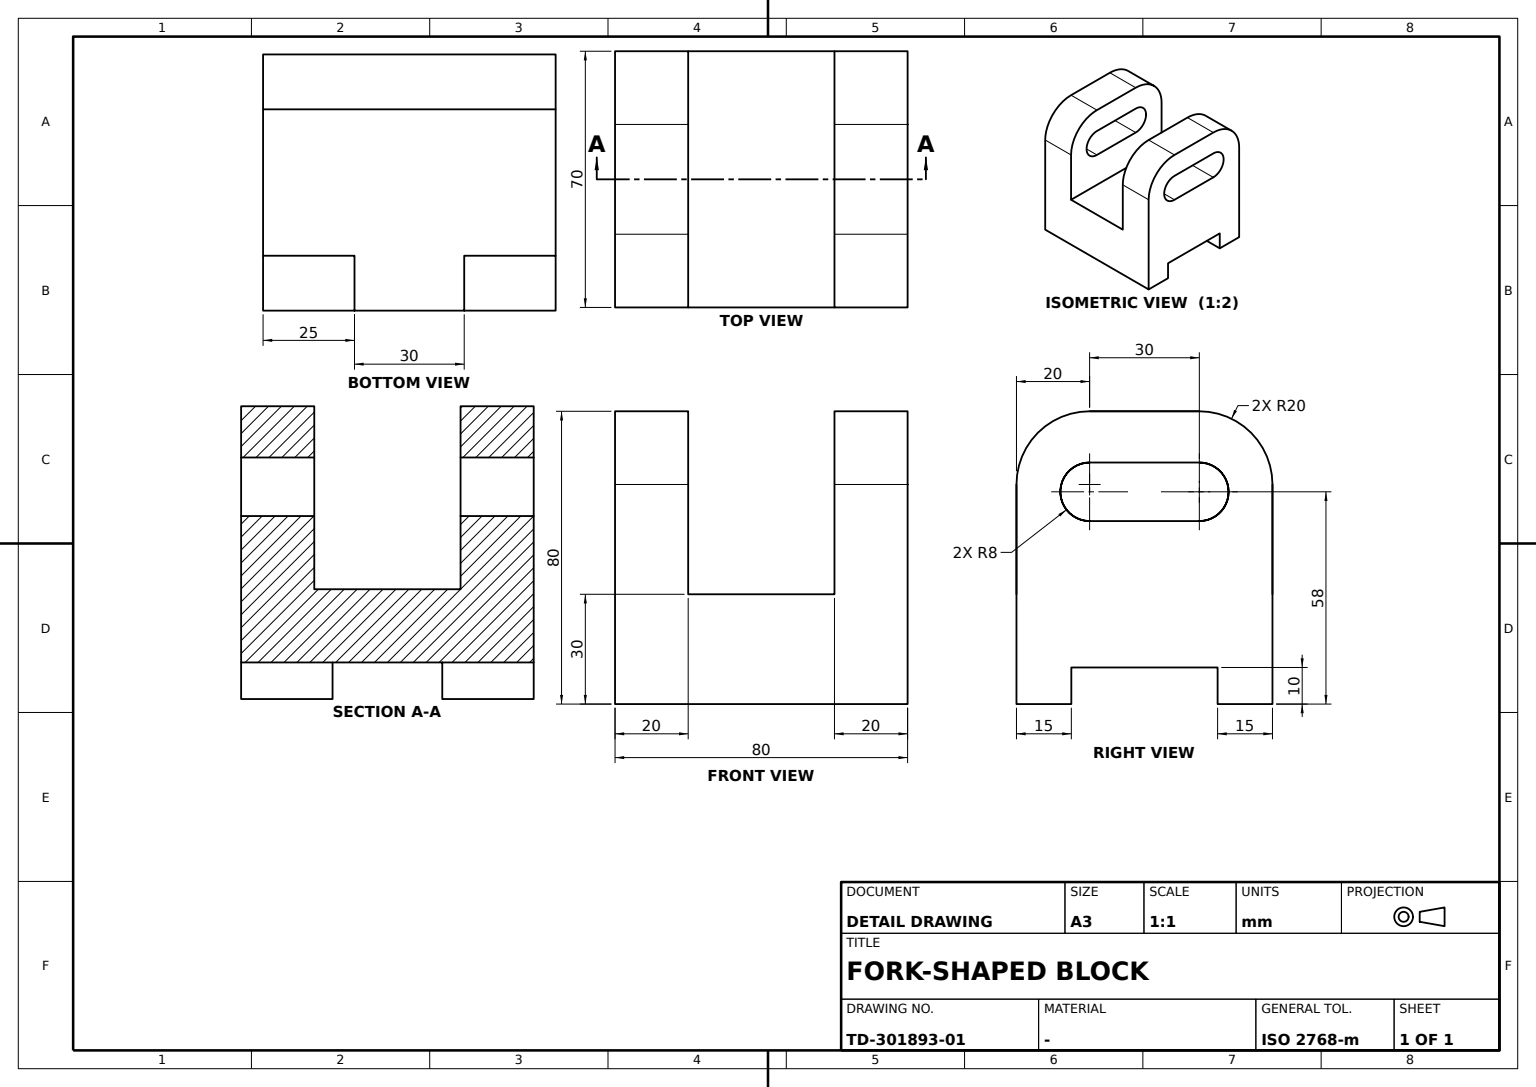
ISO-10303-21;
HEADER;
FILE_DESCRIPTION((''),'2;1');
FILE_NAME('','',(''),(''),'','','');
FILE_SCHEMA(('AUTOMOTIVE_DESIGN'));
ENDSEC;
DATA;
#1=APPLICATION_CONTEXT('');
#2=PRODUCT_CONTEXT('',#1,'mechanical');
#3=PRODUCT('','','',(#2));
#4=PRODUCT_DEFINITION_FORMATION('','',#3);
#5=PRODUCT_DEFINITION_CONTEXT('',#1,'design');
#6=PRODUCT_DEFINITION('','',#4,#5);
#7=PRODUCT_DEFINITION_SHAPE('','',#6);
#8=(LENGTH_UNIT()NAMED_UNIT(*)SI_UNIT(.MILLI.,.METRE.));
#9=(NAMED_UNIT(*)PLANE_ANGLE_UNIT()SI_UNIT($,.RADIAN.));
#10=(NAMED_UNIT(*)SI_UNIT($,.STERADIAN.)SOLID_ANGLE_UNIT());
#11=UNCERTAINTY_MEASURE_WITH_UNIT(LENGTH_MEASURE(1.E-05),#8,'distance_accuracy_value','');
#12=(GEOMETRIC_REPRESENTATION_CONTEXT(3)GLOBAL_UNCERTAINTY_ASSIGNED_CONTEXT((#11))GLOBAL_UNIT_ASSIGNED_CONTEXT((#8,#9,#10))REPRESENTATION_CONTEXT('',''));
#13=CARTESIAN_POINT('',(40.,-20.,0.));
#14=VERTEX_POINT('',#13);
#15=CARTESIAN_POINT('',(40.,20.,0.));
#16=VERTEX_POINT('',#15);
#17=CARTESIAN_POINT('',(40.,0.,0.));
#18=DIRECTION('',(0.,1.,0.));
#19=VECTOR('',#18,1000.);
#20=LINE('',#17,#19);
#21=EDGE_CURVE('',#14,#16,#20,.T.);
#22=ORIENTED_EDGE('',*,*,#21,.T.);
#23=CARTESIAN_POINT('',(40.,20.,-10.));
#24=VERTEX_POINT('',#23);
#25=CARTESIAN_POINT('',(40.,20.,-5.));
#26=DIRECTION('',(0.,0.,-1.));
#27=VECTOR('',#26,1000.);
#28=LINE('',#25,#27);
#29=EDGE_CURVE('',#16,#24,#28,.T.);
#30=ORIENTED_EDGE('',*,*,#29,.T.);
#31=CARTESIAN_POINT('',(40.,35.,-10.));
#32=VERTEX_POINT('',#31);
#33=CARTESIAN_POINT('',(40.,27.5,-10.));
#34=LINE('',#33,#19);
#35=EDGE_CURVE('',#24,#32,#34,.T.);
#36=ORIENTED_EDGE('',*,*,#35,.T.);
#37=CARTESIAN_POINT('',(40.,35.,50.));
#38=VERTEX_POINT('',#37);
#39=CARTESIAN_POINT('',(40.,35.,20.));
#40=DIRECTION('',(0.,0.,1.));
#41=VECTOR('',#40,1000.);
#42=LINE('',#39,#41);
#43=EDGE_CURVE('',#32,#38,#42,.T.);
#44=ORIENTED_EDGE('',*,*,#43,.T.);
#45=CARTESIAN_POINT('',(40.,15.,70.));
#46=VERTEX_POINT('',#45);
#47=CARTESIAN_POINT('',(40.,15.,50.));
#48=DIRECTION('',(-1.,0.,0.));
#49=AXIS2_PLACEMENT_3D('',#47,#48,#18);
#50=CIRCLE('',#49,20.);
#51=EDGE_CURVE('',#46,#38,#50,.T.);
#52=ORIENTED_EDGE('',*,*,#51,.F.);
#53=CARTESIAN_POINT('',(40.,-15.,70.));
#54=VERTEX_POINT('',#53);
#55=CARTESIAN_POINT('',(40.,0.,70.));
#56=DIRECTION('',(0.,-1.,0.));
#57=VECTOR('',#56,1000.);
#58=LINE('',#55,#57);
#59=EDGE_CURVE('',#46,#54,#58,.T.);
#60=ORIENTED_EDGE('',*,*,#59,.T.);
#61=CARTESIAN_POINT('',(40.,-35.,50.));
#62=VERTEX_POINT('',#61);
#63=CARTESIAN_POINT('',(40.,-15.,50.));
#64=AXIS2_PLACEMENT_3D('',#63,#48,#18);
#65=CIRCLE('',#64,20.);
#66=EDGE_CURVE('',#62,#54,#65,.T.);
#67=ORIENTED_EDGE('',*,*,#66,.F.);
#68=CARTESIAN_POINT('',(40.,-35.,-10.));
#69=VERTEX_POINT('',#68);
#70=CARTESIAN_POINT('',(40.,-35.,20.));
#71=LINE('',#70,#27);
#72=EDGE_CURVE('',#62,#69,#71,.T.);
#73=ORIENTED_EDGE('',*,*,#72,.T.);
#74=CARTESIAN_POINT('',(40.,-20.,-10.));
#75=VERTEX_POINT('',#74);
#76=CARTESIAN_POINT('',(40.,-27.5,-10.));
#77=LINE('',#76,#19);
#78=EDGE_CURVE('',#69,#75,#77,.T.);
#79=ORIENTED_EDGE('',*,*,#78,.T.);
#80=CARTESIAN_POINT('',(40.,-20.,-5.));
#81=LINE('',#80,#41);
#82=EDGE_CURVE('',#75,#14,#81,.T.);
#83=ORIENTED_EDGE('',*,*,#82,.T.);
#84=EDGE_LOOP('',(#22,#30,#36,#44,#52,#60,#67,#73,#79,#83));
#85=FACE_OUTER_BOUND('',#84,.T.);
#86=CARTESIAN_POINT('',(40.,-15.,56.));
#87=VERTEX_POINT('',#86);
#88=CARTESIAN_POINT('',(40.,-15.,40.));
#89=VERTEX_POINT('',#88);
#90=CARTESIAN_POINT('',(40.,-15.,48.));
#91=DIRECTION('',(1.,0.,0.));
#92=AXIS2_PLACEMENT_3D('',#90,#91,#18);
#93=CIRCLE('',#92,8.);
#94=EDGE_CURVE('',#87,#89,#93,.T.);
#95=ORIENTED_EDGE('',*,*,#94,.F.);
#96=CARTESIAN_POINT('',(40.,15.,56.));
#97=VERTEX_POINT('',#96);
#98=CARTESIAN_POINT('',(40.,0.,56.));
#99=LINE('',#98,#57);
#100=EDGE_CURVE('',#97,#87,#99,.T.);
#101=ORIENTED_EDGE('',*,*,#100,.F.);
#102=CARTESIAN_POINT('',(40.,23.,48.));
#103=VERTEX_POINT('',#102);
#104=CARTESIAN_POINT('',(40.,15.,48.));
#105=AXIS2_PLACEMENT_3D('',#104,#91,#18);
#106=CIRCLE('',#105,8.);
#107=EDGE_CURVE('',#103,#97,#106,.T.);
#108=ORIENTED_EDGE('',*,*,#107,.F.);
#109=CARTESIAN_POINT('',(40.,15.,40.));
#110=VERTEX_POINT('',#109);
#111=EDGE_CURVE('',#110,#103,#106,.T.);
#112=ORIENTED_EDGE('',*,*,#111,.F.);
#113=CARTESIAN_POINT('',(40.,0.,40.));
#114=LINE('',#113,#19);
#115=EDGE_CURVE('',#89,#110,#114,.T.);
#116=ORIENTED_EDGE('',*,*,#115,.F.);
#117=EDGE_LOOP('',(#95,#101,#108,#112,#116));
#118=FACE_BOUND('',#117,.T.);
#119=AXIS2_PLACEMENT_3D('',#17,#91,#18);
#120=PLANE('',#119);
#121=ADVANCED_FACE('',(#85,#118),#120,.T.);
#122=CARTESIAN_POINT('',(-40.,15.,70.));
#123=VERTEX_POINT('',#122);
#124=CARTESIAN_POINT('',(-20.,15.,70.));
#125=VERTEX_POINT('',#124);
#126=CARTESIAN_POINT('',(-30.,15.,70.));
#127=VECTOR('',#91,1000.);
#128=LINE('',#126,#127);
#129=EDGE_CURVE('',#123,#125,#128,.T.);
#130=ORIENTED_EDGE('',*,*,#129,.F.);
#131=CARTESIAN_POINT('',(-40.,-15.,70.));
#132=VERTEX_POINT('',#131);
#133=CARTESIAN_POINT('',(-40.,0.,70.));
#134=LINE('',#133,#57);
#135=EDGE_CURVE('',#123,#132,#134,.T.);
#136=ORIENTED_EDGE('',*,*,#135,.T.);
#137=CARTESIAN_POINT('',(-20.,-15.,70.));
#138=VERTEX_POINT('',#137);
#139=CARTESIAN_POINT('',(-30.,-15.,70.));
#140=LINE('',#139,#127);
#141=EDGE_CURVE('',#132,#138,#140,.T.);
#142=ORIENTED_EDGE('',*,*,#141,.T.);
#143=CARTESIAN_POINT('',(-20.,0.,70.));
#144=LINE('',#143,#57);
#145=EDGE_CURVE('',#125,#138,#144,.T.);
#146=ORIENTED_EDGE('',*,*,#145,.F.);
#147=EDGE_LOOP('',(#130,#136,#142,#146));
#148=FACE_OUTER_BOUND('',#147,.T.);
#149=CARTESIAN_POINT('',(0.,-35.,70.));
#150=AXIS2_PLACEMENT_3D('',#149,#26,#18);
#151=PLANE('',#150);
#152=ADVANCED_FACE('',(#148),#151,.F.);
#153=CARTESIAN_POINT('',(20.,15.,70.));
#154=VERTEX_POINT('',#153);
#155=CARTESIAN_POINT('',(30.,15.,70.));
#156=LINE('',#155,#127);
#157=EDGE_CURVE('',#154,#46,#156,.T.);
#158=ORIENTED_EDGE('',*,*,#157,.F.);
#159=CARTESIAN_POINT('',(20.,-15.,70.));
#160=VERTEX_POINT('',#159);
#161=CARTESIAN_POINT('',(20.,0.,70.));
#162=LINE('',#161,#57);
#163=EDGE_CURVE('',#154,#160,#162,.T.);
#164=ORIENTED_EDGE('',*,*,#163,.T.);
#165=CARTESIAN_POINT('',(30.,-15.,70.));
#166=LINE('',#165,#127);
#167=EDGE_CURVE('',#160,#54,#166,.T.);
#168=ORIENTED_EDGE('',*,*,#167,.T.);
#169=ORIENTED_EDGE('',*,*,#59,.F.);
#170=EDGE_LOOP('',(#158,#164,#168,#169));
#171=FACE_OUTER_BOUND('',#170,.T.);
#172=ADVANCED_FACE('',(#171),#151,.F.);
#173=CARTESIAN_POINT('',(-20.,15.,40.));
#174=VERTEX_POINT('',#173);
#175=CARTESIAN_POINT('',(-40.,15.,40.));
#176=VERTEX_POINT('',#175);
#177=CARTESIAN_POINT('',(-0.66,15.,40.));
#178=VECTOR('',#48,1000.);
#179=LINE('',#177,#178);
#180=EDGE_CURVE('',#174,#176,#179,.T.);
#181=ORIENTED_EDGE('',*,*,#180,.F.);
#182=CARTESIAN_POINT('',(-20.,23.,48.));
#183=VERTEX_POINT('',#182);
#184=CARTESIAN_POINT('',(-20.,15.,48.));
#185=AXIS2_PLACEMENT_3D('',#184,#48,#26);
#186=CIRCLE('',#185,8.);
#187=EDGE_CURVE('',#183,#174,#186,.T.);
#188=ORIENTED_EDGE('',*,*,#187,.F.);
#189=CARTESIAN_POINT('',(-40.,23.,48.));
#190=VERTEX_POINT('',#189);
#191=CARTESIAN_POINT('',(-0.66,23.,48.));
#192=LINE('',#191,#178);
#193=EDGE_CURVE('',#183,#190,#192,.T.);
#194=ORIENTED_EDGE('',*,*,#193,.T.);
#195=CARTESIAN_POINT('',(-40.,15.,48.));
#196=AXIS2_PLACEMENT_3D('',#195,#91,#18);
#197=CIRCLE('',#196,8.);
#198=EDGE_CURVE('',#176,#190,#197,.T.);
#199=ORIENTED_EDGE('',*,*,#198,.F.);
#200=EDGE_LOOP('',(#181,#188,#194,#199));
#201=FACE_OUTER_BOUND('',#200,.T.);
#202=CARTESIAN_POINT('',(-0.66,15.,48.));
#203=AXIS2_PLACEMENT_3D('',#202,#48,#18);
#204=CYLINDRICAL_SURFACE('',#203,8.);
#205=ADVANCED_FACE('',(#201),#204,.F.);
#206=CARTESIAN_POINT('',(-20.,-15.,56.));
#207=VERTEX_POINT('',#206);
#208=CARTESIAN_POINT('',(-40.,-15.,56.));
#209=VERTEX_POINT('',#208);
#210=CARTESIAN_POINT('',(-30.,-15.,56.));
#211=LINE('',#210,#178);
#212=EDGE_CURVE('',#207,#209,#211,.T.);
#213=ORIENTED_EDGE('',*,*,#212,.T.);
#214=CARTESIAN_POINT('',(-40.,15.,56.));
#215=VERTEX_POINT('',#214);
#216=CARTESIAN_POINT('',(-40.,0.,56.));
#217=LINE('',#216,#19);
#218=EDGE_CURVE('',#209,#215,#217,.T.);
#219=ORIENTED_EDGE('',*,*,#218,.T.);
#220=CARTESIAN_POINT('',(-20.,15.,56.));
#221=VERTEX_POINT('',#220);
#222=CARTESIAN_POINT('',(-0.66,15.,56.));
#223=LINE('',#222,#178);
#224=EDGE_CURVE('',#221,#215,#223,.T.);
#225=ORIENTED_EDGE('',*,*,#224,.F.);
#226=CARTESIAN_POINT('',(-20.,0.,56.));
#227=LINE('',#226,#19);
#228=EDGE_CURVE('',#207,#221,#227,.T.);
#229=ORIENTED_EDGE('',*,*,#228,.F.);
#230=EDGE_LOOP('',(#213,#219,#225,#229));
#231=FACE_OUTER_BOUND('',#230,.T.);
#232=AXIS2_PLACEMENT_3D('',#86,#40,#18);
#233=PLANE('',#232);
#234=ADVANCED_FACE('',(#231),#233,.F.);
#235=CARTESIAN_POINT('',(20.,-15.,56.));
#236=VERTEX_POINT('',#235);
#237=CARTESIAN_POINT('',(20.,-15.,40.));
#238=VERTEX_POINT('',#237);
#239=CARTESIAN_POINT('',(20.,-15.,48.));
#240=AXIS2_PLACEMENT_3D('',#239,#91,#40);
#241=CIRCLE('',#240,8.);
#242=EDGE_CURVE('',#236,#238,#241,.T.);
#243=ORIENTED_EDGE('',*,*,#242,.T.);
#244=CARTESIAN_POINT('',(20.,15.,40.));
#245=VERTEX_POINT('',#244);
#246=CARTESIAN_POINT('',(20.,0.,40.));
#247=LINE('',#246,#57);
#248=EDGE_CURVE('',#245,#238,#247,.T.);
#249=ORIENTED_EDGE('',*,*,#248,.F.);
#250=CARTESIAN_POINT('',(20.,23.,48.));
#251=VERTEX_POINT('',#250);
#252=CARTESIAN_POINT('',(20.,15.,48.));
#253=AXIS2_PLACEMENT_3D('',#252,#91,#40);
#254=CIRCLE('',#253,8.);
#255=EDGE_CURVE('',#245,#251,#254,.T.);
#256=ORIENTED_EDGE('',*,*,#255,.T.);
#257=CARTESIAN_POINT('',(20.,15.,56.));
#258=VERTEX_POINT('',#257);
#259=EDGE_CURVE('',#251,#258,#254,.T.);
#260=ORIENTED_EDGE('',*,*,#259,.T.);
#261=CARTESIAN_POINT('',(20.,0.,56.));
#262=LINE('',#261,#19);
#263=EDGE_CURVE('',#236,#258,#262,.T.);
#264=ORIENTED_EDGE('',*,*,#263,.F.);
#265=EDGE_LOOP('',(#243,#249,#256,#260,#264));
#266=FACE_BOUND('',#265,.T.);
#267=ORIENTED_EDGE('',*,*,#163,.F.);
#268=CARTESIAN_POINT('',(20.,35.,50.));
#269=VERTEX_POINT('',#268);
#270=CARTESIAN_POINT('',(20.,15.,50.));
#271=AXIS2_PLACEMENT_3D('',#270,#91,#40);
#272=CIRCLE('',#271,20.);
#273=EDGE_CURVE('',#269,#154,#272,.T.);
#274=ORIENTED_EDGE('',*,*,#273,.F.);
#275=CARTESIAN_POINT('',(20.,35.,20.));
#276=VERTEX_POINT('',#275);
#277=CARTESIAN_POINT('',(20.,35.,35.));
#278=LINE('',#277,#27);
#279=EDGE_CURVE('',#269,#276,#278,.T.);
#280=ORIENTED_EDGE('',*,*,#279,.T.);
#281=CARTESIAN_POINT('',(20.,-35.,20.));
#282=VERTEX_POINT('',#281);
#283=CARTESIAN_POINT('',(20.,0.,20.));
#284=LINE('',#283,#57);
#285=EDGE_CURVE('',#276,#282,#284,.T.);
#286=ORIENTED_EDGE('',*,*,#285,.T.);
#287=CARTESIAN_POINT('',(20.,-35.,50.));
#288=VERTEX_POINT('',#287);
#289=CARTESIAN_POINT('',(20.,-35.,35.));
#290=LINE('',#289,#41);
#291=EDGE_CURVE('',#282,#288,#290,.T.);
#292=ORIENTED_EDGE('',*,*,#291,.T.);
#293=CARTESIAN_POINT('',(20.,-15.,50.));
#294=AXIS2_PLACEMENT_3D('',#293,#91,#40);
#295=CIRCLE('',#294,20.);
#296=EDGE_CURVE('',#160,#288,#295,.T.);
#297=ORIENTED_EDGE('',*,*,#296,.F.);
#298=EDGE_LOOP('',(#267,#274,#280,#286,#292,#297));
#299=FACE_OUTER_BOUND('',#298,.T.);
#300=AXIS2_PLACEMENT_3D('',#275,#91,#40);
#301=PLANE('',#300);
#302=ADVANCED_FACE('',(#266,#299),#301,.F.);
#303=CARTESIAN_POINT('',(-20.,35.,50.));
#304=VERTEX_POINT('',#303);
#305=CARTESIAN_POINT('',(-20.,15.,50.));
#306=AXIS2_PLACEMENT_3D('',#305,#48,#26);
#307=CIRCLE('',#306,20.);
#308=EDGE_CURVE('',#125,#304,#307,.T.);
#309=ORIENTED_EDGE('',*,*,#308,.T.);
#310=CARTESIAN_POINT('',(-40.,35.,50.));
#311=VERTEX_POINT('',#310);
#312=CARTESIAN_POINT('',(-30.,35.,50.));
#313=LINE('',#312,#127);
#314=EDGE_CURVE('',#311,#304,#313,.T.);
#315=ORIENTED_EDGE('',*,*,#314,.F.);
#316=CARTESIAN_POINT('',(-40.,15.,50.));
#317=AXIS2_PLACEMENT_3D('',#316,#91,#18);
#318=CIRCLE('',#317,20.);
#319=EDGE_CURVE('',#311,#123,#318,.T.);
#320=ORIENTED_EDGE('',*,*,#319,.T.);
#321=ORIENTED_EDGE('',*,*,#129,.T.);
#322=EDGE_LOOP('',(#309,#315,#320,#321));
#323=FACE_OUTER_BOUND('',#322,.T.);
#324=CARTESIAN_POINT('',(0.,15.,50.));
#325=AXIS2_PLACEMENT_3D('',#324,#48,#40);
#326=CYLINDRICAL_SURFACE('',#325,20.);
#327=ADVANCED_FACE('',(#323),#326,.T.);
#328=CARTESIAN_POINT('',(-40.,35.,-10.));
#329=VERTEX_POINT('',#328);
#330=CARTESIAN_POINT('',(-40.,35.,20.));
#331=LINE('',#330,#41);
#332=EDGE_CURVE('',#329,#311,#331,.T.);
#333=ORIENTED_EDGE('',*,*,#332,.T.);
#334=ORIENTED_EDGE('',*,*,#314,.T.);
#335=CARTESIAN_POINT('',(-20.,35.,20.));
#336=VERTEX_POINT('',#335);
#337=CARTESIAN_POINT('',(-20.,35.,35.));
#338=LINE('',#337,#41);
#339=EDGE_CURVE('',#336,#304,#338,.T.);
#340=ORIENTED_EDGE('',*,*,#339,.F.);
#341=CARTESIAN_POINT('',(0.,35.,20.));
#342=LINE('',#341,#178);
#343=EDGE_CURVE('',#276,#336,#342,.T.);
#344=ORIENTED_EDGE('',*,*,#343,.F.);
#345=ORIENTED_EDGE('',*,*,#279,.F.);
#346=CARTESIAN_POINT('',(30.,35.,50.));
#347=LINE('',#346,#127);
#348=EDGE_CURVE('',#269,#38,#347,.T.);
#349=ORIENTED_EDGE('',*,*,#348,.T.);
#350=ORIENTED_EDGE('',*,*,#43,.F.);
#351=CARTESIAN_POINT('',(15.,35.,-10.));
#352=VERTEX_POINT('',#351);
#353=CARTESIAN_POINT('',(27.5,35.,-10.));
#354=LINE('',#353,#127);
#355=EDGE_CURVE('',#352,#32,#354,.T.);
#356=ORIENTED_EDGE('',*,*,#355,.F.);
#357=CARTESIAN_POINT('',(15.,35.,0.));
#358=VERTEX_POINT('',#357);
#359=CARTESIAN_POINT('',(15.,35.,-5.));
#360=LINE('',#359,#27);
#361=EDGE_CURVE('',#358,#352,#360,.T.);
#362=ORIENTED_EDGE('',*,*,#361,.F.);
#363=CARTESIAN_POINT('',(-15.,35.,0.));
#364=VERTEX_POINT('',#363);
#365=CARTESIAN_POINT('',(0.,35.,0.));
#366=LINE('',#365,#127);
#367=EDGE_CURVE('',#364,#358,#366,.T.);
#368=ORIENTED_EDGE('',*,*,#367,.F.);
#369=CARTESIAN_POINT('',(-15.,35.,-10.));
#370=VERTEX_POINT('',#369);
#371=CARTESIAN_POINT('',(-15.,35.,-5.));
#372=LINE('',#371,#41);
#373=EDGE_CURVE('',#370,#364,#372,.T.);
#374=ORIENTED_EDGE('',*,*,#373,.F.);
#375=CARTESIAN_POINT('',(-27.5,35.,-10.));
#376=LINE('',#375,#127);
#377=EDGE_CURVE('',#329,#370,#376,.T.);
#378=ORIENTED_EDGE('',*,*,#377,.F.);
#379=EDGE_LOOP('',(#333,#334,#340,#344,#345,#349,#350,#356,#362,#368,#374,#378));
#380=FACE_OUTER_BOUND('',#379,.T.);
#381=CARTESIAN_POINT('',(0.,35.,-10.));
#382=AXIS2_PLACEMENT_3D('',#381,#18,#40);
#383=PLANE('',#382);
#384=ADVANCED_FACE('',(#380),#383,.T.);
#385=CARTESIAN_POINT('',(-20.,-15.,40.));
#386=VERTEX_POINT('',#385);
#387=CARTESIAN_POINT('',(-40.,-15.,40.));
#388=VERTEX_POINT('',#387);
#389=CARTESIAN_POINT('',(-0.66,-15.,40.));
#390=LINE('',#389,#178);
#391=EDGE_CURVE('',#386,#388,#390,.T.);
#392=ORIENTED_EDGE('',*,*,#391,.T.);
#393=CARTESIAN_POINT('',(-40.,-15.,48.));
#394=AXIS2_PLACEMENT_3D('',#393,#91,#18);
#395=CIRCLE('',#394,8.);
#396=EDGE_CURVE('',#209,#388,#395,.T.);
#397=ORIENTED_EDGE('',*,*,#396,.F.);
#398=ORIENTED_EDGE('',*,*,#212,.F.);
#399=CARTESIAN_POINT('',(-20.,-15.,48.));
#400=AXIS2_PLACEMENT_3D('',#399,#48,#26);
#401=CIRCLE('',#400,8.);
#402=EDGE_CURVE('',#386,#207,#401,.T.);
#403=ORIENTED_EDGE('',*,*,#402,.F.);
#404=EDGE_LOOP('',(#392,#397,#398,#403));
#405=FACE_OUTER_BOUND('',#404,.T.);
#406=CARTESIAN_POINT('',(-0.66,-15.,48.));
#407=AXIS2_PLACEMENT_3D('',#406,#48,#18);
#408=CYLINDRICAL_SURFACE('',#407,8.);
#409=ADVANCED_FACE('',(#405),#408,.F.);
#410=ORIENTED_EDGE('',*,*,#377,.T.);
#411=CARTESIAN_POINT('',(-15.,20.,-10.));
#412=VERTEX_POINT('',#411);
#413=CARTESIAN_POINT('',(-15.,27.5,-10.));
#414=LINE('',#413,#57);
#415=EDGE_CURVE('',#370,#412,#414,.T.);
#416=ORIENTED_EDGE('',*,*,#415,.T.);
#417=CARTESIAN_POINT('',(-40.,20.,-10.));
#418=VERTEX_POINT('',#417);
#419=CARTESIAN_POINT('',(-27.5,20.,-10.));
#420=LINE('',#419,#127);
#421=EDGE_CURVE('',#418,#412,#420,.T.);
#422=ORIENTED_EDGE('',*,*,#421,.F.);
#423=CARTESIAN_POINT('',(-40.,27.5,-10.));
#424=LINE('',#423,#19);
#425=EDGE_CURVE('',#418,#329,#424,.T.);
#426=ORIENTED_EDGE('',*,*,#425,.T.);
#427=EDGE_LOOP('',(#410,#416,#422,#426));
#428=FACE_OUTER_BOUND('',#427,.T.);
#429=CARTESIAN_POINT('',(0.,20.,-10.));
#430=AXIS2_PLACEMENT_3D('',#429,#26,#18);
#431=PLANE('',#430);
#432=ADVANCED_FACE('',(#428),#431,.T.);
#433=ORIENTED_EDGE('',*,*,#339,.T.);
#434=ORIENTED_EDGE('',*,*,#308,.F.);
#435=ORIENTED_EDGE('',*,*,#145,.T.);
#436=CARTESIAN_POINT('',(-20.,-35.,50.));
#437=VERTEX_POINT('',#436);
#438=CARTESIAN_POINT('',(-20.,-15.,50.));
#439=AXIS2_PLACEMENT_3D('',#438,#48,#26);
#440=CIRCLE('',#439,20.);
#441=EDGE_CURVE('',#437,#138,#440,.T.);
#442=ORIENTED_EDGE('',*,*,#441,.F.);
#443=CARTESIAN_POINT('',(-20.,-35.,20.));
#444=VERTEX_POINT('',#443);
#445=CARTESIAN_POINT('',(-20.,-35.,35.));
#446=LINE('',#445,#41);
#447=EDGE_CURVE('',#444,#437,#446,.T.);
#448=ORIENTED_EDGE('',*,*,#447,.F.);
#449=CARTESIAN_POINT('',(-20.,0.,20.));
#450=LINE('',#449,#57);
#451=EDGE_CURVE('',#336,#444,#450,.T.);
#452=ORIENTED_EDGE('',*,*,#451,.F.);
#453=EDGE_LOOP('',(#433,#434,#435,#442,#448,#452));
#454=FACE_OUTER_BOUND('',#453,.T.);
#455=ORIENTED_EDGE('',*,*,#187,.T.);
#456=CARTESIAN_POINT('',(-20.,0.,40.));
#457=LINE('',#456,#57);
#458=EDGE_CURVE('',#174,#386,#457,.T.);
#459=ORIENTED_EDGE('',*,*,#458,.T.);
#460=ORIENTED_EDGE('',*,*,#402,.T.);
#461=ORIENTED_EDGE('',*,*,#228,.T.);
#462=EDGE_CURVE('',#221,#183,#186,.T.);
#463=ORIENTED_EDGE('',*,*,#462,.T.);
#464=EDGE_LOOP('',(#455,#459,#460,#461,#463));
#465=FACE_BOUND('',#464,.T.);
#466=CARTESIAN_POINT('',(-20.,35.,74.461655));
#467=AXIS2_PLACEMENT_3D('',#466,#48,#26);
#468=PLANE('',#467);
#469=ADVANCED_FACE('',(#454,#465),#468,.F.);
#470=EDGE_CURVE('',#103,#251,#192,.T.);
#471=ORIENTED_EDGE('',*,*,#470,.T.);
#472=ORIENTED_EDGE('',*,*,#255,.F.);
#473=EDGE_CURVE('',#110,#245,#179,.T.);
#474=ORIENTED_EDGE('',*,*,#473,.F.);
#475=ORIENTED_EDGE('',*,*,#111,.T.);
#476=EDGE_LOOP('',(#471,#472,#474,#475));
#477=FACE_OUTER_BOUND('',#476,.T.);
#478=ADVANCED_FACE('',(#477),#204,.F.);
#479=CARTESIAN_POINT('',(-40.,-20.,0.));
#480=VERTEX_POINT('',#479);
#481=CARTESIAN_POINT('',(-40.,20.,0.));
#482=VERTEX_POINT('',#481);
#483=CARTESIAN_POINT('',(-40.,0.,0.));
#484=LINE('',#483,#19);
#485=EDGE_CURVE('',#480,#482,#484,.T.);
#486=ORIENTED_EDGE('',*,*,#485,.T.);
#487=CARTESIAN_POINT('',(-15.,20.,0.));
#488=VERTEX_POINT('',#487);
#489=CARTESIAN_POINT('',(-27.5,20.,0.));
#490=LINE('',#489,#127);
#491=EDGE_CURVE('',#482,#488,#490,.T.);
#492=ORIENTED_EDGE('',*,*,#491,.T.);
#493=CARTESIAN_POINT('',(-15.,27.5,0.));
#494=LINE('',#493,#57);
#495=EDGE_CURVE('',#364,#488,#494,.T.);
#496=ORIENTED_EDGE('',*,*,#495,.F.);
#497=ORIENTED_EDGE('',*,*,#367,.T.);
#498=CARTESIAN_POINT('',(15.,20.,0.));
#499=VERTEX_POINT('',#498);
#500=CARTESIAN_POINT('',(15.,27.5,0.));
#501=LINE('',#500,#57);
#502=EDGE_CURVE('',#358,#499,#501,.T.);
#503=ORIENTED_EDGE('',*,*,#502,.T.);
#504=CARTESIAN_POINT('',(27.5,20.,0.));
#505=LINE('',#504,#127);
#506=EDGE_CURVE('',#499,#16,#505,.T.);
#507=ORIENTED_EDGE('',*,*,#506,.T.);
#508=ORIENTED_EDGE('',*,*,#21,.F.);
#509=CARTESIAN_POINT('',(0.,-20.,0.));
#510=LINE('',#509,#127);
#511=EDGE_CURVE('',#480,#14,#510,.T.);
#512=ORIENTED_EDGE('',*,*,#511,.F.);
#513=EDGE_LOOP('',(#486,#492,#496,#497,#503,#507,#508,#512));
#514=FACE_OUTER_BOUND('',#513,.T.);
#515=AXIS2_PLACEMENT_3D('',#509,#26,#18);
#516=PLANE('',#515);
#517=ADVANCED_FACE('',(#514),#516,.T.);
#518=EDGE_CURVE('',#89,#238,#390,.T.);
#519=ORIENTED_EDGE('',*,*,#518,.F.);
#520=ORIENTED_EDGE('',*,*,#115,.T.);
#521=ORIENTED_EDGE('',*,*,#473,.T.);
#522=ORIENTED_EDGE('',*,*,#248,.T.);
#523=EDGE_LOOP('',(#519,#520,#521,#522));
#524=FACE_OUTER_BOUND('',#523,.T.);
#525=AXIS2_PLACEMENT_3D('',#109,#26,#56);
#526=PLANE('',#525);
#527=ADVANCED_FACE('',(#524),#526,.F.);
#528=CARTESIAN_POINT('',(30.,-35.,50.));
#529=LINE('',#528,#127);
#530=EDGE_CURVE('',#288,#62,#529,.T.);
#531=ORIENTED_EDGE('',*,*,#530,.T.);
#532=ORIENTED_EDGE('',*,*,#66,.T.);
#533=ORIENTED_EDGE('',*,*,#167,.F.);
#534=ORIENTED_EDGE('',*,*,#296,.T.);
#535=EDGE_LOOP('',(#531,#532,#533,#534));
#536=FACE_OUTER_BOUND('',#535,.T.);
#537=CARTESIAN_POINT('',(0.,-15.,50.));
#538=AXIS2_PLACEMENT_3D('',#537,#48,#56);
#539=CYLINDRICAL_SURFACE('',#538,20.);
#540=ADVANCED_FACE('',(#536),#539,.T.);
#541=ORIENTED_EDGE('',*,*,#107,.T.);
#542=EDGE_CURVE('',#97,#258,#223,.T.);
#543=ORIENTED_EDGE('',*,*,#542,.T.);
#544=ORIENTED_EDGE('',*,*,#259,.F.);
#545=ORIENTED_EDGE('',*,*,#470,.F.);
#546=EDGE_LOOP('',(#541,#543,#544,#545));
#547=FACE_OUTER_BOUND('',#546,.T.);
#548=ADVANCED_FACE('',(#547),#204,.F.);
#549=CARTESIAN_POINT('',(15.,20.,-10.));
#550=VERTEX_POINT('',#549);
#551=CARTESIAN_POINT('',(27.5,20.,-10.));
#552=LINE('',#551,#127);
#553=EDGE_CURVE('',#550,#24,#552,.T.);
#554=ORIENTED_EDGE('',*,*,#553,.T.);
#555=ORIENTED_EDGE('',*,*,#29,.F.);
#556=ORIENTED_EDGE('',*,*,#506,.F.);
#557=CARTESIAN_POINT('',(15.,20.,-5.));
#558=LINE('',#557,#41);
#559=EDGE_CURVE('',#550,#499,#558,.T.);
#560=ORIENTED_EDGE('',*,*,#559,.F.);
#561=EDGE_LOOP('',(#554,#555,#556,#560));
#562=FACE_OUTER_BOUND('',#561,.T.);
#563=CARTESIAN_POINT('',(0.,20.,0.));
#564=AXIS2_PLACEMENT_3D('',#563,#56,#26);
#565=PLANE('',#564);
#566=ADVANCED_FACE('',(#562),#565,.T.);
#567=ORIENTED_EDGE('',*,*,#355,.T.);
#568=ORIENTED_EDGE('',*,*,#35,.F.);
#569=ORIENTED_EDGE('',*,*,#553,.F.);
#570=CARTESIAN_POINT('',(15.,27.5,-10.));
#571=LINE('',#570,#57);
#572=EDGE_CURVE('',#352,#550,#571,.T.);
#573=ORIENTED_EDGE('',*,*,#572,.F.);
#574=EDGE_LOOP('',(#567,#568,#569,#573));
#575=FACE_OUTER_BOUND('',#574,.T.);
#576=ADVANCED_FACE('',(#575),#431,.T.);
#577=CARTESIAN_POINT('',(-40.,-35.,-10.));
#578=VERTEX_POINT('',#577);
#579=CARTESIAN_POINT('',(0.,-35.,-10.));
#580=LINE('',#579,#127);
#581=EDGE_CURVE('',#578,#69,#580,.T.);
#582=ORIENTED_EDGE('',*,*,#581,.F.);
#583=CARTESIAN_POINT('',(-40.,-20.,-10.));
#584=VERTEX_POINT('',#583);
#585=CARTESIAN_POINT('',(-40.,-27.5,-10.));
#586=LINE('',#585,#19);
#587=EDGE_CURVE('',#578,#584,#586,.T.);
#588=ORIENTED_EDGE('',*,*,#587,.T.);
#589=CARTESIAN_POINT('',(0.,-20.,-10.));
#590=LINE('',#589,#127);
#591=EDGE_CURVE('',#584,#75,#590,.T.);
#592=ORIENTED_EDGE('',*,*,#591,.T.);
#593=ORIENTED_EDGE('',*,*,#78,.F.);
#594=EDGE_LOOP('',(#582,#588,#592,#593));
#595=FACE_OUTER_BOUND('',#594,.T.);
#596=ADVANCED_FACE('',(#595),#431,.T.);
#597=ORIENTED_EDGE('',*,*,#491,.F.);
#598=CARTESIAN_POINT('',(-40.,20.,-5.));
#599=LINE('',#598,#27);
#600=EDGE_CURVE('',#482,#418,#599,.T.);
#601=ORIENTED_EDGE('',*,*,#600,.T.);
#602=ORIENTED_EDGE('',*,*,#421,.T.);
#603=CARTESIAN_POINT('',(-15.,20.,-5.));
#604=LINE('',#603,#27);
#605=EDGE_CURVE('',#488,#412,#604,.T.);
#606=ORIENTED_EDGE('',*,*,#605,.F.);
#607=EDGE_LOOP('',(#597,#601,#602,#606));
#608=FACE_OUTER_BOUND('',#607,.T.);
#609=ADVANCED_FACE('',(#608),#565,.T.);
#610=ORIENTED_EDGE('',*,*,#591,.F.);
#611=CARTESIAN_POINT('',(-40.,-20.,-5.));
#612=LINE('',#611,#41);
#613=EDGE_CURVE('',#584,#480,#612,.T.);
#614=ORIENTED_EDGE('',*,*,#613,.T.);
#615=ORIENTED_EDGE('',*,*,#511,.T.);
#616=ORIENTED_EDGE('',*,*,#82,.F.);
#617=EDGE_LOOP('',(#610,#614,#615,#616));
#618=FACE_OUTER_BOUND('',#617,.T.);
#619=AXIS2_PLACEMENT_3D('',#509,#56,#26);
#620=PLANE('',#619);
#621=ADVANCED_FACE('',(#618),#620,.F.);
#622=ORIENTED_EDGE('',*,*,#425,.F.);
#623=ORIENTED_EDGE('',*,*,#600,.F.);
#624=ORIENTED_EDGE('',*,*,#485,.F.);
#625=ORIENTED_EDGE('',*,*,#613,.F.);
#626=ORIENTED_EDGE('',*,*,#587,.F.);
#627=CARTESIAN_POINT('',(-40.,-35.,50.));
#628=VERTEX_POINT('',#627);
#629=CARTESIAN_POINT('',(-40.,-35.,20.));
#630=LINE('',#629,#27);
#631=EDGE_CURVE('',#628,#578,#630,.T.);
#632=ORIENTED_EDGE('',*,*,#631,.F.);
#633=CARTESIAN_POINT('',(-40.,-15.,50.));
#634=AXIS2_PLACEMENT_3D('',#633,#91,#18);
#635=CIRCLE('',#634,20.);
#636=EDGE_CURVE('',#132,#628,#635,.T.);
#637=ORIENTED_EDGE('',*,*,#636,.F.);
#638=ORIENTED_EDGE('',*,*,#135,.F.);
#639=ORIENTED_EDGE('',*,*,#319,.F.);
#640=ORIENTED_EDGE('',*,*,#332,.F.);
#641=EDGE_LOOP('',(#622,#623,#624,#625,#626,#632,#637,#638,#639,#640));
#642=FACE_OUTER_BOUND('',#641,.T.);
#643=ORIENTED_EDGE('',*,*,#198,.T.);
#644=EDGE_CURVE('',#190,#215,#197,.T.);
#645=ORIENTED_EDGE('',*,*,#644,.T.);
#646=ORIENTED_EDGE('',*,*,#218,.F.);
#647=ORIENTED_EDGE('',*,*,#396,.T.);
#648=CARTESIAN_POINT('',(-40.,0.,40.));
#649=LINE('',#648,#57);
#650=EDGE_CURVE('',#176,#388,#649,.T.);
#651=ORIENTED_EDGE('',*,*,#650,.F.);
#652=EDGE_LOOP('',(#643,#645,#646,#647,#651));
#653=FACE_BOUND('',#652,.T.);
#654=AXIS2_PLACEMENT_3D('',#483,#91,#18);
#655=PLANE('',#654);
#656=ADVANCED_FACE('',(#642,#653),#655,.F.);
#657=ORIENTED_EDGE('',*,*,#373,.T.);
#658=ORIENTED_EDGE('',*,*,#495,.T.);
#659=ORIENTED_EDGE('',*,*,#605,.T.);
#660=ORIENTED_EDGE('',*,*,#415,.F.);
#661=EDGE_LOOP('',(#657,#658,#659,#660));
#662=FACE_OUTER_BOUND('',#661,.T.);
#663=AXIS2_PLACEMENT_3D('',#363,#48,#26);
#664=PLANE('',#663);
#665=ADVANCED_FACE('',(#662),#664,.F.);
#666=CARTESIAN_POINT('',(-30.,-35.,50.));
#667=LINE('',#666,#127);
#668=EDGE_CURVE('',#628,#437,#667,.T.);
#669=ORIENTED_EDGE('',*,*,#668,.F.);
#670=ORIENTED_EDGE('',*,*,#631,.T.);
#671=ORIENTED_EDGE('',*,*,#581,.T.);
#672=ORIENTED_EDGE('',*,*,#72,.F.);
#673=ORIENTED_EDGE('',*,*,#530,.F.);
#674=ORIENTED_EDGE('',*,*,#291,.F.);
#675=CARTESIAN_POINT('',(0.,-35.,20.));
#676=LINE('',#675,#127);
#677=EDGE_CURVE('',#444,#282,#676,.T.);
#678=ORIENTED_EDGE('',*,*,#677,.F.);
#679=ORIENTED_EDGE('',*,*,#447,.T.);
#680=EDGE_LOOP('',(#669,#670,#671,#672,#673,#674,#678,#679));
#681=FACE_OUTER_BOUND('',#680,.T.);
#682=AXIS2_PLACEMENT_3D('',#579,#18,#40);
#683=PLANE('',#682);
#684=ADVANCED_FACE('',(#681),#683,.F.);
#685=ORIENTED_EDGE('',*,*,#348,.F.);
#686=ORIENTED_EDGE('',*,*,#273,.T.);
#687=ORIENTED_EDGE('',*,*,#157,.T.);
#688=ORIENTED_EDGE('',*,*,#51,.T.);
#689=EDGE_LOOP('',(#685,#686,#687,#688));
#690=FACE_OUTER_BOUND('',#689,.T.);
#691=ADVANCED_FACE('',(#690),#326,.T.);
#692=ORIENTED_EDGE('',*,*,#451,.T.);
#693=ORIENTED_EDGE('',*,*,#677,.T.);
#694=ORIENTED_EDGE('',*,*,#285,.F.);
#695=ORIENTED_EDGE('',*,*,#343,.T.);
#696=EDGE_LOOP('',(#692,#693,#694,#695));
#697=FACE_OUTER_BOUND('',#696,.T.);
#698=AXIS2_PLACEMENT_3D('',#335,#26,#91);
#699=PLANE('',#698);
#700=ADVANCED_FACE('',(#697),#699,.F.);
#701=ORIENTED_EDGE('',*,*,#361,.T.);
#702=ORIENTED_EDGE('',*,*,#572,.T.);
#703=ORIENTED_EDGE('',*,*,#559,.T.);
#704=ORIENTED_EDGE('',*,*,#502,.F.);
#705=EDGE_LOOP('',(#701,#702,#703,#704));
#706=FACE_OUTER_BOUND('',#705,.T.);
#707=AXIS2_PLACEMENT_3D('',#351,#91,#40);
#708=PLANE('',#707);
#709=ADVANCED_FACE('',(#706),#708,.F.);
#710=ORIENTED_EDGE('',*,*,#668,.T.);
#711=ORIENTED_EDGE('',*,*,#441,.T.);
#712=ORIENTED_EDGE('',*,*,#141,.F.);
#713=ORIENTED_EDGE('',*,*,#636,.T.);
#714=EDGE_LOOP('',(#710,#711,#712,#713));
#715=FACE_OUTER_BOUND('',#714,.T.);
#716=ADVANCED_FACE('',(#715),#539,.T.);
#717=ORIENTED_EDGE('',*,*,#462,.F.);
#718=ORIENTED_EDGE('',*,*,#224,.T.);
#719=ORIENTED_EDGE('',*,*,#644,.F.);
#720=ORIENTED_EDGE('',*,*,#193,.F.);
#721=EDGE_LOOP('',(#717,#718,#719,#720));
#722=FACE_OUTER_BOUND('',#721,.T.);
#723=ADVANCED_FACE('',(#722),#204,.F.);
#724=ORIENTED_EDGE('',*,*,#242,.F.);
#725=CARTESIAN_POINT('',(30.,-15.,56.));
#726=LINE('',#725,#178);
#727=EDGE_CURVE('',#87,#236,#726,.T.);
#728=ORIENTED_EDGE('',*,*,#727,.F.);
#729=ORIENTED_EDGE('',*,*,#94,.T.);
#730=ORIENTED_EDGE('',*,*,#518,.T.);
#731=EDGE_LOOP('',(#724,#728,#729,#730));
#732=FACE_OUTER_BOUND('',#731,.T.);
#733=ADVANCED_FACE('',(#732),#408,.F.);
#734=ORIENTED_EDGE('',*,*,#100,.T.);
#735=ORIENTED_EDGE('',*,*,#727,.T.);
#736=ORIENTED_EDGE('',*,*,#263,.T.);
#737=ORIENTED_EDGE('',*,*,#542,.F.);
#738=EDGE_LOOP('',(#734,#735,#736,#737));
#739=FACE_OUTER_BOUND('',#738,.T.);
#740=ADVANCED_FACE('',(#739),#233,.F.);
#741=ORIENTED_EDGE('',*,*,#650,.T.);
#742=ORIENTED_EDGE('',*,*,#391,.F.);
#743=ORIENTED_EDGE('',*,*,#458,.F.);
#744=ORIENTED_EDGE('',*,*,#180,.T.);
#745=EDGE_LOOP('',(#741,#742,#743,#744));
#746=FACE_OUTER_BOUND('',#745,.T.);
#747=ADVANCED_FACE('',(#746),#526,.F.);
#748=CLOSED_SHELL('',(#121,#152,#172,#205,#234,#302,#327,#384,#409,#432,#469,#478,#517,#527,#540,#548,#566,#576,#596,#609,#621,#656,#665,#684,#691,#700,#709,#716,#723,#733,#740,#747));
#749=MANIFOLD_SOLID_BREP('',#748);
#750=ADVANCED_BREP_SHAPE_REPRESENTATION('',(#749),#12);
#751=SHAPE_DEFINITION_REPRESENTATION(#7,#750);
ENDSEC;
END-ISO-10303-21;
